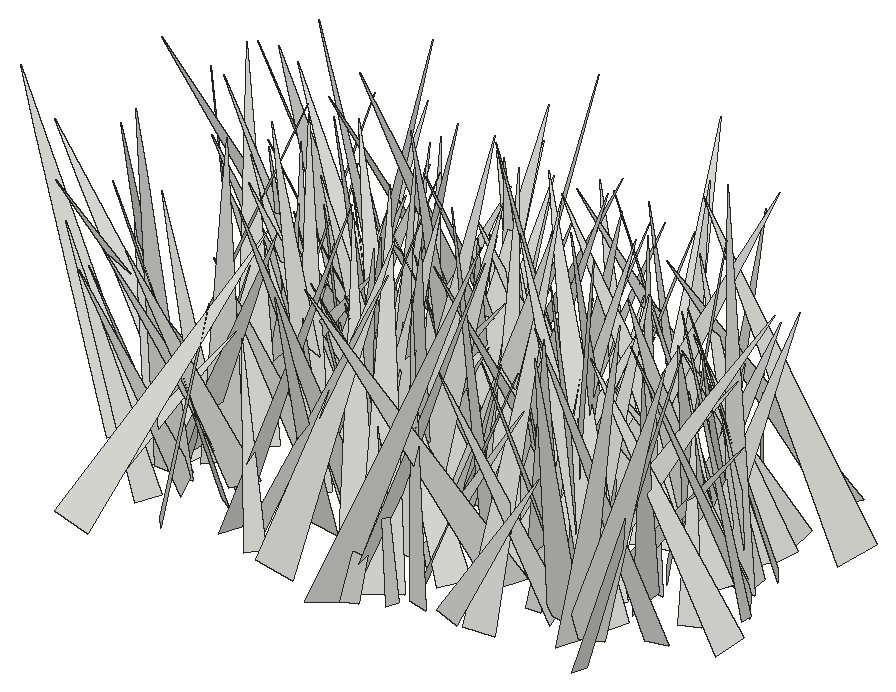
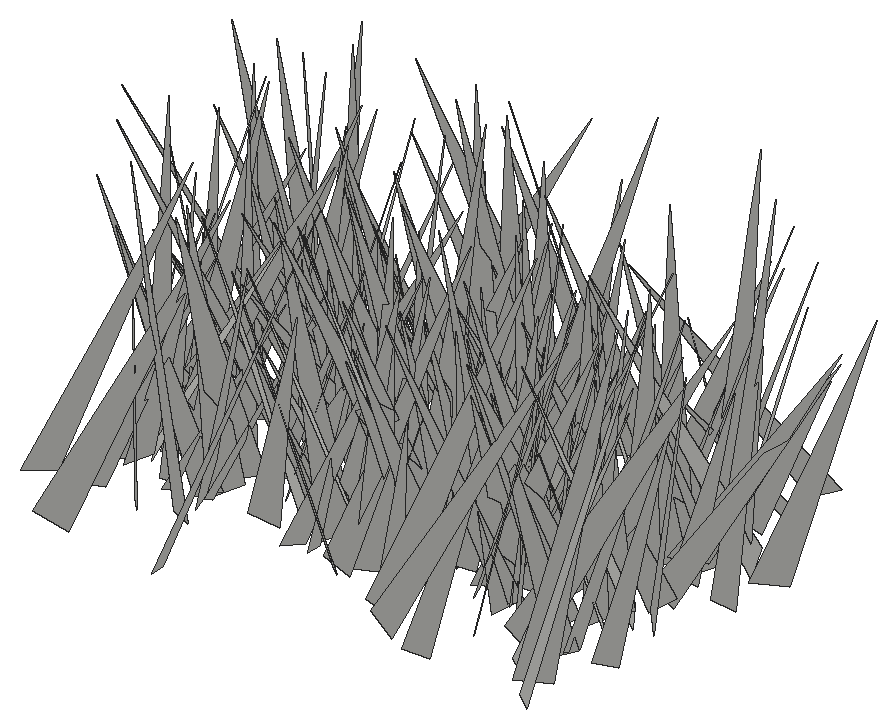
# SketchUp Ruby script. Lengths in inches.
U = 1.inch
M = Sketchup.active_model
def pt(a) = Geom::Point3d.new(a.map { |v| v * U })
def face(e, loops, mat)
  f = e.add_face(loops[0].map { |a| pt(a) })
  loops[1..].each { |l| e.add_face(l.map { |a| pt(a) }).erase! }
  f.material = f.back_material = mat if mat
  f
end
# faces: each face lists its corners as indices into pts; further lists are holes
def faces(e, pts, list, mat = nil) = list.each { |f| face(e, (f[0].is_a?(Array) ? f : [f]).map { |l| l.map { |i| pts[i] } }, mat) }
# xy, xz, yz: faces in a plane at the given z, y or x. An outline is a flat list of corners, or four numbers for a rectangle; further outlines are holes
def ring(l) = l.size == 4 ? [[l[0], l[1]], [l[2], l[1]], [l[2], l[3]], [l[0], l[3]]] : l.each_slice(2).to_a
def flat(e, list, mat, &to3) = list.each { |f| face(e, (f[0].is_a?(Array) ? f : [f]).map { |l| ring(l).map { |u, v| to3.(u, v) } }, mat) }
def xy(e, z, list, mat = nil) = flat(e, list, mat) { |x, y| [x, y, z] }
def xz(e, y, list, mat = nil) = flat(e, list, mat) { |x, z| [x, y, z] }
def yz(e, x, list, mat = nil) = flat(e, list, mat) { |y, z| [x, y, z] }
def lines(e, pts, list) = list.each { |a, b| e.add_line(pt(pts[a]), pt(pts[b])) }
# prism: a flat outline (further loops are holes) pulled along v
def prism(e, loops, v, mat = nil)
  f = face(e, loops, mat); d = Geom::Vector3d.new(v.map { |x| x * U })
  f.pushpull(f.normal.samedirection?(d) ? d.length : -d.length)
end
def box(e, o, s, mat = nil) = prism(e, [[o, [o[0] + s[0], o[1], o[2]], [o[0] + s[0], o[1] + s[1], o[2]], [o[0], o[1] + s[1], o[2]]]], [0, 0, s[2]], mat)
def at(x, y, z, deg = 0) = Geom::Transformation.translation(pt([x, y, z])) * Geom::Transformation.rotation(ORIGIN, Z_AXIS, deg.degrees)
def axes(o, x, y, z) = Geom::Transformation.new([*x, 0, *y, 0, *z, 0, *pt(o).to_a, 1])
def part(name) = M.definitions.add(name)
# library, detail: a bought-in or finely detailed component or shape, given as its bounding box
def library(name, o, s) = part(name).tap { |d| box(d.entities, o, s) }
def detail(e, o, s) = box(e.add_group.entities, o, s)
def put(e, d, t, mat = nil) = e.add_instance(d, t).tap { |i| i.material = mat if mat }
def group(e, t, mat = nil) = e.add_group.tap { |g| g.transformation = t; g.material = mat if mat }.entities
root = M.entities
c1 = part("fur_instance\#9")
p = [[0.8125,0,1.79],[0.67,-0.02,1.48],[0,-0.11,0],[0,0.11,0]]
faces(c1.entities,p,[[0,1,2,3]])
put(root,c1,axes([458.41,60.53,-21.86],[-5.34659,-1.99732,0.9572],[-1.60106,5.21354,1.93576],[1.5304,-1.52357,5.36919]))
put(root,c1,axes([472.33,58.41,-21.66],[1.50617,-3.93782,1.16858],[-3.70084,-0.76096,2.20573],[1.78207,1.74788,3.59301]))
put(root,c1,axes([467.86,56.82,-21.86],[7.81962,-2.04899,1.63917],[-2.46618,-7.49875,2.3913],[-0.8962,2.75717,7.72182]))
put(root,c1,axes([457.11,55.375,-21.66],[-1.44675,6.62808,0.1342],[5.91861,1.35324,-3.03008],[2.98656,0.529,6.06986]))
put(root,c1,axes([459.44,57.69,-21.86],[3.19373,2.97376,0.94617],[2.91746,-3.32577,0.60507],[-1.10768,-0.18543,4.3217]))
put(root,c1,axes([463.52,58.16,-21.86],[-3.55756,1.9012,0.49829],[1.88183,3.59228,-0.2708],[0.56709,0.00632,4.02461]))
put(root,c1,axes([464.95,57.51,-21.86],[-0.40245,7.17423,1.83924],[7.10701,0.89237,-1.92572],[2.08393,-1.65784,6.92265]))
put(root,c1,axes([462.5,59.63,-21.86],[6.41393,4.45568,0.74677],[4.39818,-5.86174,-2.80093],[1.0328,-2.70854,7.29015]))
put(root,c1,axes([475.74,61.13,-21.86],[0.50064,-7.21064,0.91051],[-7.21991,-0.3887,0.89157],[0.83387,0.96363,7.17281]))
put(root,c1,axes([469.97,58.18,-21.86],[-4.02809,-0.22088,0.67447],[-0.39433,3.92835,-1.06856],[0.59008,1.11738,3.89005]))
put(root,c1,axes([468.86,57.03,-21.66],[-4.41847,1.33903,1.10997],[0.76139,4.21375,-2.05244],[1.56375,1.73183,4.13562]))
put(root,c1,axes([472.6,61.78,-21.66],[1.75618,-7.20882,1.45322],[-6.25973,-2.24953,-3.59425],[-3.85938,0.3683,6.49097]))
put(root,c1,axes([464.45,61.1,-21.86],[-0.34138,-6.1128,0.75859],[-6.1403,0.39794,0.44341],[0.48829,0.7305,6.10625]))
put(root,c1,axes([459.45,62.29,-21.86],[-5.6995,-3.45113,0.56108],[-3.05969,5.44221,2.39374],[1.69215,-1.78365,6.21808]))
put(root,c1,axes([466.45,61.41,-21.86],[-0.98604,-7.77609,1.14314],[-7.75331,0.77346,-1.42635],[-1.28859,1.29646,7.70749]))
put(root,c1,axes([470.74,58.69,-21.86],[2.01081,5.29668,2.07869],[5.40677,-2.46554,1.0522],[-1.77275,-1.51176,5.56697]))
put(root,c1,axes([456.25,57.85,-21.66],[-0.23722,4.19444,0.05409],[3.55446,0.22976,-2.22834],[2.22756,0.08005,3.56147]))
put(root,c1,axes([460.31,61.6,-21.66],[2.04194,-5.37013,1.21962],[-4.97283,-2.35693,-2.05211],[-2.36574,0.31918,5.36625]))
put(root,c1,axes([456.87,61.59,-21.86],[-3.71629,-3.62879,0.54604],[-3.4741,3.72939,1.13989],[1.18191,-0.44788,5.0675]))
put(root,c1,axes([458,58.77,-21.86],[-1.87407,5.07403,0.37598],[4.58214,1.50899,2.47512],[-2.21159,-1.17322,4.80954]))
put(root,c1,axes([475.15,61.4,-21.86],[-5.60277,-1.40853,0.55452],[-1.25772,5.51462,1.29985],[0.84237,-1.13469,5.62898]))
put(root,c1,axes([468.0625,58.57,-21.86],[-5.00326,5.02156,1.24961],[5.08502,5.09325,-0.10752],[0.95924,-0.80806,7.08781]))
put(root,c1,axes([457.51,60.9,-21.86],[-0.06707,-7.91469,2.47451],[-8.29222,0.04381,-0.08466],[-0.06773,2.47503,7.91452]))
put(root,c1,axes([468.37,58.11,-21.86],[6.99612,0.8962,1.32294],[0.53893,-6.91662,1.83548],[-1.5043,1.69005,6.81028]))
put(root,c1,axes([469.15,58.51,-21.86],[-4.81371,6.17541,1.55135],[6.27572,4.93015,-0.15223],[1.07597,-1.1279,7.82843]))
put(root,c1,axes([460.37,60.35,-21.86],[-4.54723,-4.75664,0.92618],[-4.80738,4.26788,-1.68375],[-0.61038,1.82216,6.36144]))
put(root,c1,axes([477.09,60.54,-21.86],[5.41416,-4.66063,0.97473],[-4.76032,-5.26587,1.26282],[0.1044,1.59183,7.03135]))
put(root,c1,axes([476.88,60.16,-21.86],[6.67765,-1.57713,2.05629],[-1.75682,-6.93326,0.38749],[-1.90506,0.86558,6.85042]))
put(root,c1,axes([462.05,58.5625,-21.66],[6.79493,0.95964,1.40947],[0.56386,-6.72962,1.86359],[-1.60922,1.6941,6.60447]))
put(root,c1,axes([478.59,58.39,-21.66],[5.94248,2.0649,1.47313],[1.51819,-5.90154,2.14801],[-2.032,1.62942,5.91295]))
put(root,c1,axes([473.33,62.99,-21.86],[1.38948,-7.3294,0.52561],[-7.22169,-1.26322,1.47599],[1.35779,0.7818,7.31247]))
put(root,c1,axes([474.26,63.14,-21.86],[-4.28945,-4.51982,0.83876],[-4.25056,4.33652,1.63064],[1.75072,-0.54543,6.01408]))
put(root,c1,axes([466.57,60.39,-21.86],[-0.74897,7.24815,2.93985],[7.55595,1.43371,-1.60981],[2.0214,-2.6736,7.1067]))
put(root,c1,axes([479.34,62.02,-21.86],[-2.01567,-6.30283,1.43527],[-6.28052,1.55369,-1.99742],[-1.52993,1.92587,6.30864]))
put(root,c1,axes([468.86,61.45,-21.66],[3.3459,3.39415,0.39754],[3.18536,-2.89609,-2.08314],[1.23764,-1.72213,4.2867]))
put(root,c1,axes([470.95,60.58,-21.66],[-3.6214,4.75768,0.36392],[4.63089,3.39426,1.70771],[-1.15013,-1.31374,5.73008]))
put(root,c1,axes([467.2,62.83,-21.86],[-2.33347,-4.94017,0.88075],[-4.99474,2.38012,0.11709],[0.48332,0.74554,5.4623]))
put(root,c1,axes([456.74,61.13,-21.86],[-2.06507,4.56305,1.47225],[4.79287,1.92061,0.77009],[-0.13147,-1.65628,4.94903]))
put(root,c1,axes([464.35,63.04,-21.86],[-4.28655,1.17606,1.86698],[1.8295,4.17484,1.57066],[1.23356,-2.10497,4.15821]))
put(root,c1,axes([466.17,63.875,-21.86],[5.44226,-5.9088,0.26751],[-5.91243,-5.44486,0.01623],[-0.16928,0.20777,8.03317]))
put(root,c1,axes([457.14,62.24,-21.86],[5.86888,-2.59714,0.14419],[-2.59865,-5.83866,0.60558],[0.11385,0.61201,6.38922]))
put(root,c1,axes([473.9375,58.32,-21.66],[1.42623,8.08681,0.06748],[7.92603,-1.41139,1.61901],[-1.60595,0.21606,8.05043]))
put(root,c1,axes([454.77,64.3,-21.66],[-2.27672,-7.40144,1.23154],[-7.29478,2.48469,1.44709],[1.75622,0.72557,7.60728]))
put(root,c1,axes([477.21,64.04,-21.86],[6.59264,-0.88288,1.14982],[-0.53637,-6.4595,-1.88457],[-1.3468,-1.74924,6.37893]))
put(root,c1,axes([477.1,61.2,-21.86],[-4.32916,0.66549,1.27706],[0.40908,4.44763,-0.93094],[1.38073,0.76884,4.27993]))
put(root,c1,axes([458.37,62.67,-21.86],[-4.86484,4.13925,3.64162],[4.78109,5.5858,0.03796],[2.74517,-2.39309,6.38738]))
put(root,c1,axes([476.33,61.95,-21.86],[-5.98871,-2.33617,1.80164],[-2.60473,6.10133,-0.74665],[1.38529,1.37273,6.38474]))
put(root,c1,axes([454.45,61.99,-21.66],[-5.80896,4.38047,0.69826],[4.41604,5.60261,1.59041],[-0.41794,-1.68592,7.09952]))
put(root,c1,axes([469.88,60.08,-21.86],[3.89032,1.8987,0.46131],[1.51623,-3.58179,1.95558],[-1.23244,1.58688,3.86204]))
put(root,c1,axes([477.36,61.7,-21.86],[-7.32829,2.58062,0.59876],[2.60966,7.33524,0.32553],[0.45582,-0.50666,7.76257]))
put(root,c1,axes([474.51,62.85,-21.86],[5.33637,4.77614,2.80857],[5.34994,-5.45601,-0.88678],[-1.44141,-2.56842,7.10647]))
put(root,c1,axes([471.3,62.43,-21.86],[-6.68963,-2.36331,2.10659],[-2.62997,6.88987,-0.62215],[1.76244,1.31094,7.06748]))
put(root,c1,axes([457.82,62.625,-21.66],[-5.05806,4.73106,0.08976],[4.36112,4.60989,2.7757],[-1.83619,-2.08349,6.34527]))
put(root,c1,axes([481.63,63.43,-21.86],[-6.11827,1.22354,0.04324],[1.20265,5.96505,1.37981],[-0.22923,-1.36132,6.08493]))
put(root,c1,axes([469.25,62.22,-21.86],[-1.66623,3.3763,0.05798],[2.90925,1.40249,1.93607],[-1.71436,-0.9015,3.22914]))
put(root,c1,axes([457.53,61.53,-21.86],[3.79033,1.52401,0.8214],[1.29616,-3.80865,1.0854],[-1.14773,0.73179,3.93842]))
put(root,c1,axes([463.29,64.46,-21.66],[0.26156,-6.27199,1.2943],[-6.21893,0.06053,1.55008],[1.52905,1.31908,6.08306]))
put(root,c1,axes([456.97,65.15,-21.66],[-0.73144,-5.99959,0.26703],[-5.39662,0.53861,-2.681],[-2.63493,0.56233,5.41685]))
put(root,c1,axes([473.3125,63.65,-21.86],[-2.39364,-3.13142,1.17859],[-3.27618,2.48779,-0.04385],[0.67935,0.9641,3.94124]))
put(root,c1,axes([460.79,64.88,-21.86],[0.69444,-4.60057,1.02449],[-4.36557,-1.0182,-1.61314],[-1.77671,0.70364,4.36409]))
put(root,c1,axes([474.25,61.12,-21.86],[2.45384,5.3856,0.3895],[5.06414,-2.44383,1.88676],[-1.87372,0.44803,5.60947]))
put(root,c1,axes([475.48,63.8,-21.86],[-3.37227,-0.8607,0.92289],[-0.91034,3.4828,-0.07828],[0.87397,0.30665,3.4795]))
put(root,c1,axes([480.21,66.42,-21.86],[-5.39374,-4.42373,0.73063],[-4.15874,5.36317,1.77113],[1.67573,-0.92879,6.74722]))
put(root,c1,axes([467.85,64.77,-21.86],[3.73133,2.74864,1.27928],[3.02044,-3.19509,-1.94493],[0.26177,-2.31318,4.20655]))
put(root,c1,axes([457.3125,63.375,-21.86],[-1.60239,4.56784,1.22355],[4.62571,1.24567,1.40748],[-0.98238,-1.58525,4.63161]))
put(root,c1,axes([455.82,61.0625,-21.66],[6.85876,3.23862,0.41321],[3.02392,-6.66397,2.03701],[-1.23097,1.67477,7.30628]))
put(root,c1,axes([467.32,62.65,-21.66],[5.50822,-3.47682,2.75588],[-4.25576,-5.38219,1.71589],[-1.25366,2.99458,6.28367]))
put(root,c1,axes([461.15,64.73,-21.86],[3.4639,-0.21189,1.20284],[0.06017,-3.58323,-0.80448],[-1.21988,-0.7784,3.37584]))
put(root,c1,axes([462.18,63.91,-21.86],[-6.35948,3.06032,1.72749],[3.24757,6.48259,0.47123],[1.34279,-1.18457,7.04176]))
put(root,c1,axes([474.48,62.74,-21.86],[3.56611,7.00423,0.23479],[6.50816,-3.2121,-3.02618],[2.59966,-1.56674,7.25387]))
put(root,c1,axes([479.5,63.75,-21.86],[-1.55614,3.71904,0.91385],[3.82438,1.56093,0.15988],[0.20123,-0.90564,4.0283]))
put(root,c1,axes([462.2,63.94,-21.86],[-2.19401,4.08598,0.64459],[3.98986,1.89782,1.55038],[-1.09165,-1.27572,4.37096]))
put(root,c1,axes([465.19,64,-21.86],[4.12414,-1.44643,0.07491],[-1.4095,-3.95608,1.21201],[0.33327,1.1677,4.19901]))
put(root,c1,axes([475.61,63.66,-21.66],[3.92135,-2.35365,0.03406],[-2.05535,-3.39138,2.27856],[1.14733,1.96892,3.96545]))
put(root,c1,axes([467.82,60.95,-21.66],[-7.05102,3.6652,1.50452],[2.87345,6.84526,-3.20935],[2.72774,2.26338,7.26985]))
put(root,c1,axes([473.01,66.26,-21.66],[-1.63485,-6.2778,0.46595],[-5.97391,1.39539,-2.16005],[-1.98499,0.97094,6.117]))
put(root,c1,axes([476.04,62.99,-21.86],[-6.13421,5.52562,0.24546],[5.52788,6.11218,0.5523],[-0.18784,-0.57446,8.23747]))
put(root,c1,axes([462.51,62.875,-21.86],[-6.55915,2.85076,0.80174],[2.70921,6.56329,-1.17278],[1.19574,0.76707,7.05506]))
put(root,c1,axes([474.25,63.75,-21.86],[-0.35457,5.93898,1.63328],[6.05839,0.63143,-0.98081],[1.11129,-1.54746,5.86815]))
put(root,c1,axes([465.6,65.97,-21.86],[-2.21504,-4.22644,0.02495],[-4.06696,2.12371,-1.31133],[-1.15036,0.62998,4.58799]))
put(root,c1,axes([471.79,62.86,-21.66],[1.01067,5.88602,0.15693],[5.68933,-0.93518,-1.56469],[1.51703,-0.41415,5.76354]))
put(root,c1,axes([473.3125,67.01,-21.66],[-6.68782,-2.79113,3.18251],[-2.04813,7.34131,2.13449],[3.70459,-0.98003,6.92541]))
put(root,c1,axes([456.73,65.41,-21.86],[2.58062,-5.27777,0.62862],[-4.46822,-1.77579,3.43383],[2.87837,1.97518,4.76689]))
put(root,c1,axes([461.7,66.83,-21.86],[6.23542,-1.61716,0.46655],[-1.48447,-6.12774,-1.40019],[-0.79324,-1.24458,6.2877]))
put(root,c1,axes([477.67,67.57,-21.86],[5.45366,-4.66647,1.60556],[-4.21255,-5.64853,-2.10822],[-2.57063,-0.64365,6.86103]))
put(root,c1,axes([462.15,65.36,-21.86],[-5.34119,3.3335,0.99515],[3.47843,5.14626,1.43085],[0.05516,-1.74201,6.13133]))
put(root,c1,axes([471.48,64.8,-21.86],[2.86437,6.58912,2.04567],[6.83224,-2.40073,-1.83379],[0.96006,-2.57407,6.94682]))
put(root,c1,axes([464.09,68.08,-21.66],[4.06405,-3.6671,0.18626],[-3.28339,-3.75381,-2.26428],[-1.64366,-1.56845,4.98369]))
put(root,c1,axes([469.9,63.56,-21.86],[7.57177,-0.43303,1.80554],[-0.88332,-7.50835,1.90355],[-1.63317,2.05334,7.34137]))
put(root,c1,axes([473.14,63.8,-21.86],[-3.67286,3.55796,0.5072],[3.52102,3.70767,-0.51167],[0.72023,0.01818,5.08794]))
put(root,c1,axes([466.76,66.84,-21.86],[-1.19832,-8.06423,2.00487],[-8.30399,1.23724,0.01324],[0.30817,1.98109,8.15276]))
put(root,c1,axes([476.96,67.54,-21.66],[6.03542,-2.39463,0.80521],[-2.12324,-5.9379,-1.74415],[-1.3691,-1.34759,6.25448]))
put(root,c1,axes([462.76,62.57,-21.66],[5.4592,3.52611,0.65952],[3.05756,-5.20187,2.50265],[-1.87611,1.78282,5.99776]))
put(root,c1,axes([470.1,66.09,-21.86],[3.7544,-3.60472,1.46029],[-3.77286,-3.86843,0.15082],[-0.94444,1.12393,5.20257]))
put(root,c1,axes([467.47,65.6875,-21.66],[2.98572,-5.88102,1.99527],[-6.13329,-2.44486,1.97166],[0.97482,2.63026,6.29392]))
put(root,c1,axes([471.61,63.28,-21.66],[-2.11402,4.56513,0.60738],[3.84978,2.11854,-2.52378],[2.52756,0.59144,4.35202]))
put(root,c1,axes([476.72,64.97,-21.86],[1.78909,6.44129,2.50482],[6.73985,-2.19865,0.83993],[-1.52927,-2.15428,6.63216]))
put(root,c1,axes([457.5,66.95,-21.66],[0.9975,-5.62203,0.93729],[-5.55991,-0.75041,1.41599],[1.25425,1.14473,5.53148]))
put(root,c1,axes([464.08,66.13,-21.86],[-5.02266,3.34128,1.54054],[3.64584,4.87057,1.32283],[0.49523,-1.96924,5.88569]))
put(root,c1,axes([461.49,67.58,-21.86],[3.15853,-4.87453,2.05329],[-4.28659,-3.76007,-2.33247],[-3.09874,0.23284,5.31949]))
put(root,c1,axes([462.39,65.46,-21.66],[3.74419,-3.98525,0.35569],[-3.51637,-3.04515,2.89653],[1.90889,2.20738,4.63803]))
put(root,c1,axes([458.74,64.3,-21.86],[-6.24341,4.5177,1.05822],[4.50521,6.32678,-0.4296],[1.11019,-0.26807,7.69449]))
put(root,c1,axes([461.56,66.66,-21.86],[-3.89073,-3.2521,0.98713],[-3.3181,3.95947,-0.03367],[0.73538,0.65937,5.07078]))
put(root,c1,axes([470.96,63.36,-21.66],[-6.61706,2.95045,0.41304],[2.75432,6.44194,-1.89112],[1.13554,1.56763,6.99387]))
put(root,c1,axes([464.9375,65.86,-21.86],[4.30722,-1.10997,0.82887],[-1.21703,-4.32511,0.53238],[-0.66174,0.72977,4.41597]))
put(root,c1,axes([462.18,66.68,-21.86],[-7.66892,-1.90839,0.15613],[-1.91216,7.66661,-0.21311],[0.09999,0.24454,7.89993]))
put(root,c1,axes([481.03,65.17,-21.66],[-5.46466,-2.11839,0.66349],[-2.21236,5.05235,-2.09036],[-0.18243,2.18553,5.47545]))
put(root,c1,axes([467.67,64.97,-21.66],[6.41211,-0.61612,1.30158],[-0.93497,-6.2989,1.62436],[-1.09524,1.77006,6.23347]))
put(root,c1,axes([458.65,67.22,-21.86],[-5.67591,-0.59927,2.29984],[-0.30227,6.08824,0.84044],[2.35734,-0.66225,5.64524]))
put(root,c1,axes([473.96,66.44,-21.86],[-5.15429,0.32159,0.0951],[0.32057,5.15491,-0.05731],[0.09848,0.05128,5.164]))
put(root,c1,axes([473.07,66.12,-21.66],[3.04424,4.32162,0.01521],[3.85535,-2.70735,-2.39804],[1.95268,-1.39208,4.71097]))
put(root,c1,axes([478.96,66.59,-21.66],[-4.49913,6.58347,1.21187],[6.27218,3.63575,3.53468],[-2.33889,-2.91414,7.14775]))
put(root,c1,axes([472.97,66.98,-21.86],[-7.3033,-3.33888,1.09507],[-3.45877,7.27632,-0.88176],[0.61989,1.26191,7.98178]))
put(root,c1,axes([461.24,68.49,-21.86],[6.14406,2.36607,3.59044],[3.36505,-6.54408,-1.44586],[-2.67694,-2.79567,6.42319]))
put(root,c1,axes([465.47,68.84,-21.86],[5.23311,-3.59302,0.50013],[-3.53385,-5.24745,-0.7222],[-0.81967,-0.31597,6.30664]))
put(root,c1,axes([464.02,65.63,-21.86],[-5.31881,4.24046,0.31909],[4.24772,5.322,0.07866],[0.20039,-0.26047,6.80184]))
put(root,c1,axes([464.98,64.14,-21.86],[1.87355,6.48838,0.26131],[6.01197,-1.83596,2.48253],[-2.45429,0.45575,6.28063]))
put(root,c1,axes([479.52,67.74,-21.86],[-3.67755,-0.2078,1.11626],[-0.0694,3.8179,0.48208],[1.13331,-0.4405,3.65173]))
put(root,c1,axes([463.2,66.69,-21.86],[1.59622,5.71911,2.00108],[6.0184,-1.73595,0.16062],[-0.70101,-1.88115,5.93551]))
put(root,c1,axes([476.47,66.2,-21.86],[5.20843,4.28763,1.83578],[4.29945,-5.48037,0.60158],[-1.80791,-0.68076,6.71935]))
put(root,c1,axes([474.51,69.86,-21.66],[-4.21387,-1.59887,0.24339],[-1.27519,3.70248,2.24451],[0.99474,-2.02671,3.90836]))
put(root,c1,axes([457.23,70.14,-21.86],[-6.16239,-2.08969,1.53365],[-1.42213,6.03269,2.50561],[2.16712,-1.98337,6.00531]))
put(root,c1,axes([471.39,65.95,-21.86],[3.38601,2.0667,0.33408],[1.88033,-3.28152,1.24252],[-0.92044,0.89903,3.76728]))
put(root,c1,axes([476.59,69.71,-21.66],[-1.94792,-5.41513,0.85515],[-5.11405,2.12183,1.78705],[1.97517,0.15336,5.47032]))
put(root,c1,axes([478.5625,66.65,-21.86],[-0.98772,3.5916,0.11089],[3.35733,0.88143,1.35606],[-1.28071,-0.45933,3.46934]))
put(root,c1,axes([456.02,66.93,-21.66],[-4.69579,-3.74143,2.09942],[-4.25802,4.44495,-1.60248],[0.52452,2.58851,5.78625]))
put(root,c1,axes([466.47,65.74,-21.86],[-3.17908,7.18759,1.82609],[7.05927,3.54175,-1.65087],[2.27218,-0.9472,7.68392]))
put(root,c1,axes([479.19,67.09,-21.86],[1.25442,7.48082,2.76942],[7.81491,-1.71475,1.09211],[-1.59984,-2.51056,7.50623]))
put(root,c1,axes([464.62,67.62,-21.86],[4.97792,-1.2009,1.19397],[-1.36113,-5.04298,0.6026],[-1.0075,0.87956,5.08515]))
put(root,c1,axes([477.46,66.97,-21.86],[0.44188,5.84269,1.52194],[5.83939,-0.02571,-1.59672],[1.53457,-1.58458,5.63763]))
put(root,c1,axes([466.94,69.91,-21.86],[1.62052,-5.44249,0.65001],[-5.43307,-1.68456,-0.55967],[-0.72449,0.45919,5.65098]))
put(root,c1,axes([479.66,68.74,-21.86],[-4.41159,-3.54695,0.73212],[-3.61607,4.3782,-0.57829],[0.20221,0.91078,5.63104]))
put(root,c1,axes([465.4,65.89,-21.86],[1.09357,6.43106,0.77169],[6.11568,-1.28298,2.02542],[-2.13365,-0.38127,6.20097]))
put(root,c1,axes([464.28,69.57,-21.86],[-3.11173,-3.4795,0.92655],[-3.33661,3.24675,0.98692],[1.3537,0.0043,4.56244]))
put(root,c1,axes([457.89,67.94,-21.86],[-4.75498,1.70819,1.94206],[1.76287,5.11453,-0.18234],[1.89256,-0.47231,5.04921]))
put(root,c1,axes([476.19,70.21,-21.66],[-4.14982,-0.72477,0.23143],[-0.53834,3.70403,1.94686],[0.53763,-1.88541,3.73578]))
put(root,c1,axes([465.37,70.16,-21.86],[-3.18461,-4.17271,0.10236],[-4.17132,3.18622,0.10881],[0.1486,0.01532,5.24799]))
put(root,c1,axes([467.9375,70.59,-21.86],[-1.54524,-6.7658,0.51217],[-6.71547,1.44992,-1.10738],[-0.96994,0.74015,6.85109]))
put(root,c1,axes([469.35,68.74,-21.86],[6.16664,-2.56617,1.31423],[-2.70082,-6.22755,0.51287],[-1.00896,0.98602,6.65955]))
put(root,c1,axes([472.15,66.83,-21.66],[2.96543,7.80813,0.73471],[7.53088,-2.61577,-2.59693],[2.18919,-1.57838,7.9383]))
put(root,c1,axes([461.15,69.0625,-21.86],[7.358,-0.55238,1.16955],[-0.51092,-7.44716,-0.30295],[-1.18825,-0.21839,7.37248]))
put(root,c1,axes([455.375,70.48,-21.66],[3.46395,-3.11936,0.86631],[-2.7787,-3.51575,-1.54862],[-1.66124,-0.62369,4.39672]))
put(root,c1,axes([465.95,67.25,-21.86],[7.28902,-0.71217,0.57332],[-0.83779,-7.04721,1.89755],[-0.36604,1.94818,7.07364]))
put(root,c1,axes([459.1,70.81,-21.86],[-1.39061,-8.04384,0.83594],[-7.45661,0.94696,-3.29214],[-3.13068,1.31752,7.46987]))
put(root,c1,axes([466.47,66.5,-21.86],[-1.14169,6.19263,0.48775],[6.13199,1.20279,-0.91762],[0.99261,-0.30768,6.22978]))
put(root,c1,axes([459.74,70.26,-21.86],[-3.39488,-3.98848,1.56761],[-3.7052,3.73666,1.48306],[2.15333,0.14147,5.02331]))
put(root,c1,axes([458.86,69.3,-21.86],[-2.76326,-3.0585,1.38467],[-3.15346,2.97986,0.28892],[1.15213,0.82059,4.11176]))
put(root,c1,axes([478.91,67.47,-21.86],[-6.97142,-3.26118,0.0354],[-2.96258,6.29742,-3.28677],[-1.3637,2.99072,6.9594]))
put(root,c1,axes([470.22,70.32,-21.86],[-6.07615,0.58264,0.90457],[0.83184,5.83413,1.82981],[0.68247,-1.92372,5.8233]))
put(root,c1,axes([462.67,66.59,-21.66],[-4.26385,3.34064,0.29483],[3.15748,4.15963,-1.468],[1.13011,0.98225,5.21395]))
put(root,c1,axes([469.64,67.72,-21.86],[-3.01404,5.97197,0.86388],[5.95256,2.78442,1.51964],[-0.98886,-1.44144,6.51457]))
put(root,c1,axes([479.28,69.65,-21.66],[-4.32688,2.05759,1.06704],[2.30248,4.07514,1.47851],[0.2661,-1.80382,4.55737]))
put(root,c1,axes([457.04,66.72,-21.86],[5.18703,3.91751,0.7095],[3.72248,-5.18551,1.41748],[-1.41191,0.72053,6.34373]))
put(root,c1,axes([466.62,70,-21.86],[2.81734,-6.20209,1.85033],[-6.41792,-2.93797,-0.07572],[-0.83667,1.65211,6.81158]))
put(root,c1,axes([460.77,66.41,-21.66],[7.1916,2.06862,2.54607],[1.20326,-7.37063,2.58975],[-3.05186,1.96861,7.0208]))
put(root,c1,axes([469.4,70.1,-21.86],[-4.25466,-1.2014,1.34721],[-0.93808,4.41863,0.97784],[1.54219,-0.62673,4.31153]))
put(root,c1,axes([462.35,68.47,-21.66],[-5.71185,4.45959,0.23835],[4.39877,5.55102,1.55146],[-0.77178,-1.36683,7.07857]))
put(root,c1,axes([468.09,69.42,-21.86],[-1.30466,-3.28465,1.2487],[-3.51229,1.2605,-0.354],[0.10971,1.29326,3.5165]))
put(root,c1,axes([469.07,67.81,-21.86],[4.58247,4.01128,0.43645],[4.00699,-4.60163,0.22113],[-0.47421,-0.12046,6.08609]))
put(root,c1,axes([471.45,67.71,-21.86],[-0.73079,4.32054,0.1844],[4.30671,0.74406,-0.36572],[0.39156,-0.12013,4.36662]))
put(root,c1,axes([462.77,68.45,-21.66],[-7.75285,-2.01113,0.68817],[-2.11722,7.53738,-1.82488],[0.1887,1.94117,7.79879]))
put(root,c1,axes([478.69,71.36,-21.86],[-4.86866,0.51762,1.11395],[0.97098,4.41082,2.19421],[0.75234,-2.34296,4.3769]))
put(root,c1,axes([470.61,68.85,-21.86],[5.68273,3.19615,0.64935],[3.24559,-5.67036,-0.49352],[-0.32122,-0.74969,6.50117]))
put(root,c1,axes([475.02,69.3,-21.86],[2.29321,-4.71361,1.70331],[-4.8602,-1.63403,2.02152],[1.22385,2.34308,4.83635]))
put(root,c1,axes([459.85,66.8125,-21.86],[-5.19171,3.73852,1.55221],[3.028,5.26206,-2.54592],[2.68647,1.29382,5.8693]))
put(root,c1,axes([478.64,68.83,-21.86],[-5.80582,1.67481,0.45332],[1.66732,5.82342,-0.1609],[0.48013,0.02943,6.04042]))
put(root,c1,axes([458.46,68.95,-21.66],[4.54931,-2.96003,1.24819],[-3.21199,-4.22741,1.68171],[-0.05363,2.09362,5.16041]))
put(root,c1,axes([467.13,69.42,-21.86],[-3.69691,-1.68274,0.52652],[-1.75981,3.59718,-0.85985],[0.10916,1.00233,3.96981]))
put(root,c1,axes([460.98,68.98,-21.66],[0.71966,5.69009,1.64056],[5.43341,0.02279,-2.46251],[2.35511,-1.79132,5.17987]))
put(root,c1,axes([466.73,67.24,-21.66],[-5.00496,1.9066,1.35129],[1.19771,4.83542,-2.3864],[2.00664,1.8693,4.79477]))
put(root,c1,axes([457.36,68.11,-21.86],[3.04107,3.48011,0.59696],[3.3547,-3.09349,0.94446],[-1.10161,0.1866,4.52408]))
put(root,c1,axes([467.38,66.6,-21.66],[5.51307,6.12337,0.96272],[5.81555,-5.55551,2.03274],[-2.14519,0.67601,7.98483]))
put(root,c1,axes([457.28,70.49,-21.86],[2.87453,-4.20489,0.68169],[-4.14129,-2.56592,1.63539],[0.99777,1.46412,4.82385]))
put(root,c1,axes([474.62,68.73,-21.86],[-5.70861,3.53079,2.01517],[3.32922,6.05385,-1.17592],[2.33318,0.00055,6.60847]))
put(root,c1,axes([464.28,72.44,-21.66],[-0.7633,-7.78268,1.04828],[-7.63293,0.4877,-1.93706],[-1.84592,1.20152,7.57632]))
put(root,c1,axes([461.03,71.04,-21.86],[-4.42725,-2.60663,1.07476],[-2.66002,4.52485,0.01676],[0.93485,0.53053,5.13759]))
put(root,c1,axes([466.13,69.61,-21.86],[-3.60805,2.068,0.36238],[2.05277,3.62596,-0.25393],[0.44056,0.04128,4.15092]))
put(root,c1,axes([458.07,72.3,-21.86],[-3.26059,-4.43586,0.10579],[-4.43536,3.26207,0.0775],[0.12511,0.03932,5.50476]))
put(root,c1,axes([474.9375,69.65,-21.86],[-6.0397,-1.24718,1.08354],[-1.47294,5.92489,-1.39057],[0.74831,1.59618,6.00831]))
put(root,c1,axes([461.57,73.9,-21.86],[4.70734,-3.12135,0.14145],[-2.64852,-4.12178,-2.81392],[-1.65776,-2.27815,4.89732]))
put(root,c1,axes([464.94,68.27,-21.86],[-1.71935,6.00909,0.23442],[5.94835,1.73522,-0.85232],[0.8839,0.01135,6.19184]))
put(root,c1,axes([480.98,71.75,-21.86],[-7.28796,2.50197,0.93453],[2.66483,6.99355,2.0583],[0.17855,-2.25345,7.42547]))
put(root,c1,axes([474.8,67.52,-21.86],[-4.41357,6.91206,0.00056],[6.86097,4.38103,-0.99489],[0.83882,0.53496,8.14041]))
put(root,c1,axes([474.7,71.27,-21.86],[-2.78435,-5.66723,3.39056],[-5.97834,3.72634,1.319],[2.80584,2.3158,6.17497]))
put(root,c1,axes([467.8125,70.85,-21.86],[4.35224,4.23695,0.82253],[4.28263,-4.09432,-1.57033],[0.53605,-1.68972,5.86752]))
put(root,c1,axes([456.875,72.82,-21.86],[4.91943,-4.73173,2.30235],[-4.40019,-5.42749,-1.75256],[-2.8859,0.2095,6.59686]))
put(root,c1,axes([471.95,69.85,-21.66],[-1.56415,5.71782,0.81541],[5.62888,1.31989,1.54221],[-1.29382,-1.17019,5.72377]))
put(root,c1,axes([463.7,73.24,-21.66],[-2.5504,-6.61055,0.06946],[-6.29815,2.40698,-2.17909],[-2.00934,0.84606,6.74207]))
put(root,c1,axes([478.24,74.51,-21.86],[2.18391,-6.70079,0.42323],[-6.08063,-2.16263,-2.86325],[-2.84706,-0.52116,6.43986]))
put(root,c1,axes([476.64,71.54,-21.86],[2.87799,2.64757,1.74089],[2.94858,-3.09885,-0.16173],[-1.16026,-1.30792,3.90721]))
put(root,c1,axes([472.91,74.91,-21.86],[-6.78403,-3.28205,0.63683],[-2.89291,6.48484,2.60352],[1.67585,-2.09175,7.07224]))
put(root,c1,axes([456.03,74.49,-21.66],[-4.76858,-5.56642,0.65425],[-5.40433,4.79429,1.40014],[1.48534,-0.42682,7.19472]))
